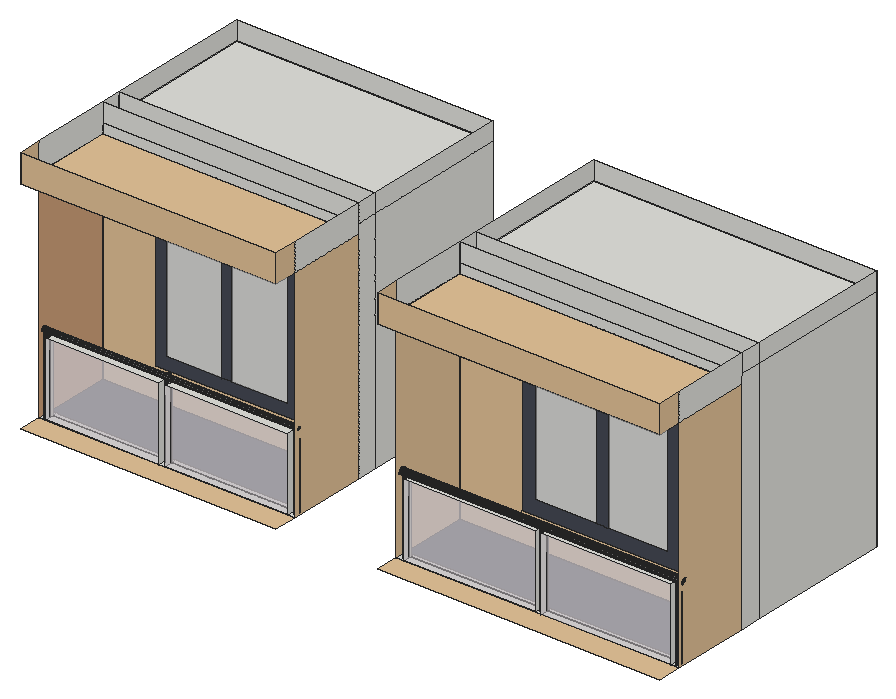
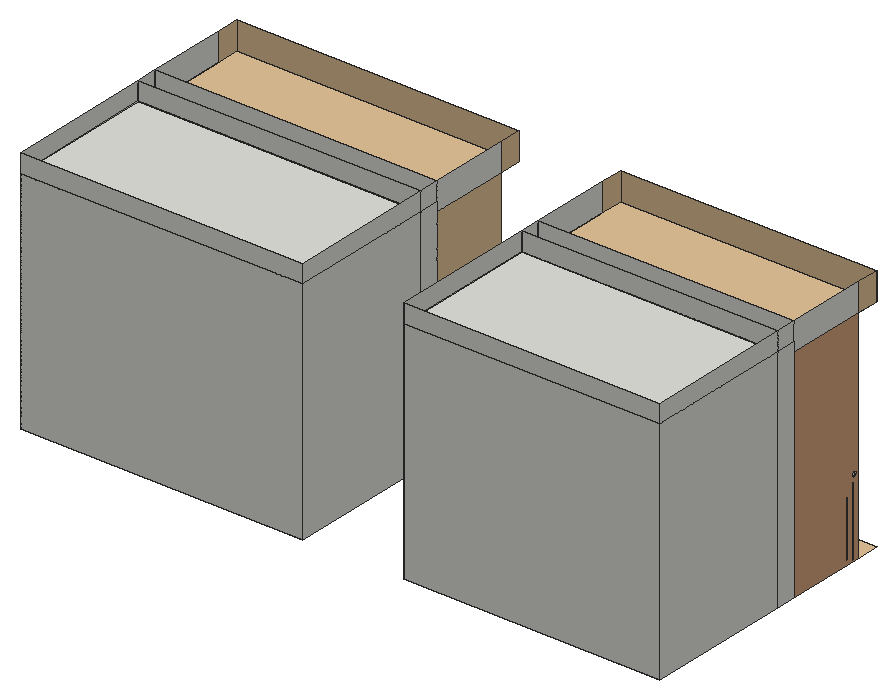
# SketchUp Ruby script. Lengths in inches.
U = 1.inch
M = Sketchup.active_model
def pt(a) = Geom::Point3d.new(a.map { |v| v * U })
def face(e, loops, mat)
  f = e.add_face(loops[0].map { |a| pt(a) })
  loops[1..].each { |l| e.add_face(l.map { |a| pt(a) }).erase! }
  f.material = f.back_material = mat if mat
  f
end
# faces: each face lists its corners as indices into pts; further lists are holes
def faces(e, pts, list, mat = nil) = list.each { |f| face(e, (f[0].is_a?(Array) ? f : [f]).map { |l| l.map { |i| pts[i] } }, mat) }
# xy, xz, yz: faces in a plane at the given z, y or x. An outline is a flat list of corners, or four numbers for a rectangle; further outlines are holes
def ring(l) = l.size == 4 ? [[l[0], l[1]], [l[2], l[1]], [l[2], l[3]], [l[0], l[3]]] : l.each_slice(2).to_a
def flat(e, list, mat, &to3) = list.each { |f| face(e, (f[0].is_a?(Array) ? f : [f]).map { |l| ring(l).map { |u, v| to3.(u, v) } }, mat) }
def xy(e, z, list, mat = nil) = flat(e, list, mat) { |x, y| [x, y, z] }
def xz(e, y, list, mat = nil) = flat(e, list, mat) { |x, z| [x, y, z] }
def yz(e, x, list, mat = nil) = flat(e, list, mat) { |y, z| [x, y, z] }
def lines(e, pts, list) = list.each { |a, b| e.add_line(pt(pts[a]), pt(pts[b])) }
# prism: a flat outline (further loops are holes) pulled along v
def prism(e, loops, v, mat = nil)
  f = face(e, loops, mat); d = Geom::Vector3d.new(v.map { |x| x * U })
  f.pushpull(f.normal.samedirection?(d) ? d.length : -d.length)
end
def box(e, o, s, mat = nil) = prism(e, [[o, [o[0] + s[0], o[1], o[2]], [o[0] + s[0], o[1] + s[1], o[2]], [o[0], o[1] + s[1], o[2]]]], [0, 0, s[2]], mat)
def at(x, y, z, deg = 0) = Geom::Transformation.translation(pt([x, y, z])) * Geom::Transformation.rotation(ORIGIN, Z_AXIS, deg.degrees)
def axes(o, x, y, z) = Geom::Transformation.new([*x, 0, *y, 0, *z, 0, *pt(o).to_a, 1])
def part(name) = M.definitions.add(name)
# library, detail: a bought-in or finely detailed component or shape, given as its bounding box
def library(name, o, s) = part(name).tap { |d| box(d.entities, o, s) }
def detail(e, o, s) = box(e.add_group.entities, o, s)
def put(e, d, t, mat = nil) = e.add_instance(d, t).tap { |i| i.material = mat if mat }
def group(e, t, mat = nil) = e.add_group.tap { |g| g.transformation = t; g.material = mat if mat }.entities
root = M.entities
M.materials.add("[0035_Tan]").color = [229, 196, 153]
M.materials.add("[Cladding Siding Tan]").color = [211, 164, 124]
M.materials.add("[Color M05]").color = [114, 114, 114]
M.materials.add("[Formica Laminate Dark]").color = [70, 74, 84]
M.materials.add("[Suede Blue]").color = [50, 57, 70]
M.materials.add("[Translucent Glass Gray]").color = [214, 214, 214]
M.materials["[Translucent Glass Gray]"].alpha = 0.5
M.materials.add("[Translucent Glass Safety]1").color = [244, 237, 242]
M.materials["[Translucent Glass Safety]1"].alpha = 0.5
xy(root,524.8125,[[[225.05,423.82,230.94,436.91],[228.4375,426.02,227.84,426.1,227.28,426.33,226.8,426.7,226.4375,427.18,226.2,427.73,226.125,428.33,226.2,428.93,226.4375,429.49,226.8,429.97,227.28,430.33,227.84,430.57,228.4375,430.64,229.04,430.57,229.59,430.33,230.07,429.97,230.44,429.49,230.67,428.93,230.75,428.33,230.67,427.73,230.44,427.18,230.07,426.7,229.59,426.33,229.04,426.1]],[230.94,423.82,335.79,431.96],[[335.79,423.82,340.97,436.91],[338.4375,428.08,337.84,428.16,337.28,428.39,336.8,428.76,336.4375,429.24,336.2,429.8,336.125,430.39,336.2,430.99,336.4375,431.55,336.8,432.03,337.28,432.4,337.84,432.63,338.4375,432.71,339.04,432.63,339.59,432.4,340.07,432.03,340.44,431.55,340.67,430.99,340.75,430.39,340.67,429.8,340.44,429.24,340.07,428.76,339.59,428.39,339.04,428.16]],[340.97,423.82,454.47,431.96],[[454.47,423.82,460.75,436.91],[457,428.08,456.4,428.16,455.84,428.39,455.37,428.76,455,429.24,454.77,429.8,454.6875,430.39,454.77,430.99,455,431.55,455.37,432.03,455.84,432.4,456.4,432.63,457,432.71,457.6,432.63,458.16,432.4,458.64,432.03,459,431.55,459.23,430.99,459.3125,430.39,459.23,429.8,459,429.24,458.64,428.76,458.16,428.39,457.6,428.16]],
  [[553.875,423.82,561.125,435],[558.4,426.88,557.77,426.96,557.1875,427.2,556.68,427.59,556.29,428.1,556.05,428.68,555.97,429.32,556.05,429.95,556.29,430.53,556.68,431.04,557.1875,431.43,557.77,431.67,558.4,431.75,559.04,431.67,559.625,431.43,560.13,431.04,560.52,430.53,560.76,429.95,560.84,429.32,560.76,428.68,560.52,428.1,560.13,427.59,559.625,427.2,559.04,426.96]],[561.125,423.82,682.3125,431.3],[[682.3125,423.82,687.5625,435],[684.97,426.88,684.34,426.96,683.75,427.2,683.24,427.59,682.86,428.1,682.61,428.68,682.53,429.32,682.61,429.95,682.86,430.53,683.24,431.04,683.75,431.43,684.34,431.67,684.97,431.75,685.6,431.67,686.1875,431.43,686.69,431.04,687.08,430.53,687.32,429.95,687.4,429.32,687.32,428.68,687.08,428.1,686.69,427.59,686.1875,427.2,685.6,426.96]],[687.5625,423.82,807.1,431.3],[[807.1,423.82,814,435],[809.9,426.88,809.27,426.96,808.6875,427.2,808.18,427.59,807.79,428.1,807.55,428.68,807.47,429.32,807.55,429.95,807.79,430.53,808.18,431.04,808.6875,431.43,809.27,431.67,809.9,431.75,810.54,431.67,811.125,431.43,811.63,431.04,812.02,430.53,812.26,429.95,812.34,429.32,812.26,428.68,812.02,428.1,811.63,427.59,811.125,427.2,810.54,426.96]],
  [228.4375,426.02,227.84,426.1,227.28,426.33,226.8,426.7,226.4375,427.18,226.2,427.73,226.125,428.33,226.2,428.93,226.4375,429.49,226.8,429.97,227.28,430.33,227.84,430.57,228.4375,430.64,229.04,430.57,229.59,430.33,230.07,429.97,230.44,429.49,230.67,428.93,230.75,428.33,230.67,427.73,230.44,427.18,230.07,426.7,229.59,426.33,229.04,426.1],[558.4,426.88,557.77,426.96,557.1875,427.2,556.68,427.59,556.29,428.1,556.05,428.68,555.97,429.32,556.05,429.95,556.29,430.53,556.68,431.04,557.1875,431.43,557.77,431.67,558.4,431.75,559.04,431.67,559.625,431.43,560.13,431.04,560.52,430.53,560.76,429.95,560.84,429.32,560.76,428.68,560.52,428.1,560.13,427.59,559.625,427.2,559.04,426.96],[684.97,426.88,684.34,426.96,683.75,427.2,683.24,427.59,682.86,428.1,682.61,428.68,682.53,429.32,682.61,429.95,682.86,430.53,683.24,431.04,683.75,431.43,684.34,431.67,684.97,431.75,685.6,431.67,686.1875,431.43,686.69,431.04,687.08,430.53,687.32,429.95,687.4,429.32,687.32,428.68,687.08,428.1,686.69,427.59,686.1875,427.2,685.6,426.96],[809.9,426.88,809.27,426.96,808.6875,427.2,808.18,427.59,807.79,428.1,807.55,428.68,807.47,429.32,807.55,429.95,807.79,430.53,808.18,431.04,808.6875,431.43,809.27,431.67,809.9,431.75,810.54,431.67,811.125,431.43,811.63,431.04,812.02,430.53,812.26,429.95,812.34,429.32,812.26,428.68,812.02,428.1,811.63,427.59,811.125,427.2,810.54,426.96],[338.4375,428.08,337.84,428.16,337.28,428.39,336.8,428.76,336.4375,429.24,336.2,429.8,336.125,430.39,336.2,430.99,336.4375,431.55,336.8,432.03,337.28,432.4,337.84,432.63,338.4375,432.71,339.04,432.63,339.59,432.4,340.07,432.03,340.44,431.55,340.67,430.99,340.75,430.39,340.67,429.8,340.44,429.24,340.07,428.76,339.59,428.39,339.04,428.16],
  [457,428.08,456.4,428.16,455.84,428.39,455.37,428.76,455,429.24,454.77,429.8,454.6875,430.39,454.77,430.99,455,431.55,455.37,432.03,455.84,432.4,456.4,432.63,457,432.71,457.6,432.63,458.16,432.4,458.64,432.03,459,431.55,459.23,430.99,459.3125,430.39,459.23,429.8,459,429.24,458.64,428.76,458.16,428.39,457.6,428.16],[561.125,431.3,682.3125,435],[687.5625,431.3,807.1,435],[230.94,431.96,335.79,436.91],[340.97,431.96,454.47,436.91],
  [225.05,496.86,460.75,515.85],[553.875,496.86,814,515.85],[225.05,515.85,460.75,651.39],[553.875,515.85,814,651.39]])
xy(root,524.8125,[[225.05,402.38,460.75,423.82],[553.875,402.38,814,423.82]],"[0035_Tan]")
xy(root,524.8125,[[553.875,435,814,496.86],[225.05,436.91,460.75,496.86]],"[Suede Blue]")
xy(root,592.1875,[[230.94,423.82,335.79,431.96],[340.97,423.82,454.47,431.96],[561.125,423.82,682.3125,431.3],[687.5625,423.82,807.1,431.3]])
xy(root,593.42,[[684.97,426.88,685.6,426.96,686.1875,427.2,686.69,427.59,687.08,428.1,687.32,428.68,687.4,429.32,687.32,429.95,687.08,430.53,686.69,431.04,686.1875,431.43,685.6,431.67,684.97,431.75,684.34,431.67,683.75,431.43,683.24,431.04,682.86,430.53,682.61,429.95,682.53,429.32,682.61,428.68,682.86,428.1,683.24,427.59,683.75,427.2,684.34,426.96]])
xy(root,594.16,[[558.4,426.88,559.04,426.96,559.625,427.2,560.13,427.59,560.52,428.1,560.76,428.68,560.84,429.32,560.76,429.95,560.52,430.53,560.13,431.04,559.625,431.43,559.04,431.67,558.4,431.75,557.77,431.67,557.1875,431.43,556.68,431.04,556.29,430.53,556.05,429.95,555.97,429.32,556.05,428.68,556.29,428.1,556.68,427.59,557.1875,427.2,557.77,426.96],[809.9,426.88,810.54,426.96,811.125,427.2,811.63,427.59,812.02,428.1,812.26,428.68,812.34,429.32,812.26,429.95,812.02,430.53,811.63,431.04,811.125,431.43,810.54,431.67,809.9,431.75,809.27,431.67,808.6875,431.43,808.18,431.04,807.79,430.53,807.55,429.95,807.47,429.32,807.55,428.68,807.79,428.1,808.18,427.59,808.6875,427.2,809.27,426.96]])
xy(root,594.5625,[[457,428.08,457.6,428.16,458.16,428.39,458.64,428.76,459,429.24,459.23,429.8,459.3125,430.39,459.23,430.99,459,431.55,458.64,432.03,458.16,432.4,457.6,432.63,457,432.71,456.4,432.63,455.84,432.4,455.37,432.03,455,431.55,454.77,430.99,454.6875,430.39,454.77,429.8,455,429.24,455.37,428.76,455.84,428.39,456.4,428.16]])
xy(root,596.5625,[[228.4375,426.02,229.04,426.1,229.59,426.33,230.07,426.7,230.44,427.18,230.67,427.73,230.75,428.33,230.67,428.93,230.44,429.49,230.07,429.97,229.59,430.33,229.04,430.57,228.4375,430.64,227.84,430.57,227.28,430.33,226.8,429.97,226.4375,429.49,226.2,428.93,226.125,428.33,226.2,427.73,226.4375,427.18,226.8,426.7,227.28,426.33,227.84,426.1]])
xy(root,597.06,[[338.4375,428.08,339.04,428.16,339.59,428.39,340.07,428.76,340.44,429.24,340.67,429.8,340.74,430.35,336.13,430.35,336.2,429.8,336.4375,429.24,336.8,428.76,337.28,428.39,337.84,428.16],[336.13,430.35,340.74,430.35,340.75,430.39,340.67,430.99,340.44,431.55,340.07,432.03,339.59,432.4,339.04,432.63,338.4375,432.71,337.84,432.63,337.28,432.4,336.8,432.03,336.4375,431.55,336.2,430.99,336.125,430.39]])
xy(root,727.0625,[[225.05,402.38,460.75,496.86],[553.875,402.38,814,496.86]],"[0035_Tan]")
xy(root,735.5,[[225.05,496.86,460.75,515.85],[553.875,496.86,814,515.85],[225.05,515.85,460.75,651.39],[553.875,515.85,814,651.39]])
xz(root,402.38,[[225.05,727.0625,460.75,752.6875],[553.875,727.0625,814,752.6875]],"[0035_Tan]")
xz(root,423.82,[[230.94,524.8125,335.79,592.1875],[340.97,524.8125,454.47,592.1875],[561.125,524.8125,682.3125,592.1875],[687.5625,524.8125,807.1,592.1875]],"[Translucent Glass Safety]1")
xz(root,431.3,[[561.125,524.8125,682.3125,592.1875],[687.5625,524.8125,807.1,592.1875]],"[Translucent Glass Safety]1")
xz(root,431.96,[[230.94,524.8125,335.79,592.1875],[340.97,524.8125,454.47,592.1875]],"[Translucent Glass Safety]1")
xz(root,496.86,[[225.05,727.0625,460.75,735.5],[553.875,727.0625,814,735.5],[225.05,735.5,460.75,752.6875],[553.875,735.5,814,752.6875]])
xz(root,496.86,[[[225.05,524.8125,460.75,727.0625],[273.85,552.86,406.72,707.17]],[[553.875,524.8125,814,727.0625],[611.02,551.65,759.09,708.4]]],"[0035_Tan]")
xz(root,496.86,[[[611.02,551.65,759.09,708.4],[624.18,564.81,745.92,695.24]],[[273.85,552.86,406.72,707.17],[284.63,563.64,395.95,696.39]],[335.36,563.64,344.53,696.39],[679.95,564.81,691.15,695.24]],"[Formica Laminate Dark]")
xz(root,496.86,[[284.63,563.64,335.36,696.39],[344.53,563.64,395.95,696.39],[624.18,564.81,679.95,695.24],[691.15,564.81,745.92,695.24]],"[Translucent Glass Gray]")
xz(root,515.85,[[225.05,524.8125,460.75,735.5],[553.875,524.8125,814,735.5],[225.05,735.5,460.75,752.6875],[553.875,735.5,814,752.6875]])
xz(root,651.39,[[225.05,524.8125,460.75,735.5],[553.875,524.8125,814,735.5],[225.05,735.5,460.75,752.6875],[553.875,735.5,814,752.6875]])
yz(root,225.05,[[496.86,524.8125,515.85,735.5],[515.85,524.8125,651.39,735.5],[428.41,594.54,427.9,594.61,427.41,594.81,427,595.13,426.68,595.54,426.48,596.02,426.41,596.54,426.48,597.06,426.68,597.54,427,597.96,427.41,598.27,427.9,598.47,428.41,598.54,428.93,598.47,429.41,598.27,429.83,597.96,430.15,597.54,430.35,597.06,430.41,596.54,430.35,596.02,430.15,595.54,429.83,595.13,429.41,594.81,428.93,594.61],[423.82,727.0625,496.86,752.6875],[496.86,735.5,515.85,752.6875],
  [515.85,735.5,651.39,752.6875]])
yz(root,225.05,[[402.38,727.0625,423.82,752.6875]],"[0035_Tan]")
yz(root,225.05,[[[423.82,524.8125,496.86,727.0625],[428.41,594.54,427.9,594.61,427.41,594.81,427,595.13,426.68,595.54,426.48,596.02,426.41,596.54,426.48,597.06,426.68,597.54,427,597.96,427.41,598.27,427.9,598.47,428.41,598.54,428.93,598.47,429.41,598.27,429.83,597.96,430.15,597.54,430.35,597.06,430.41,596.54,430.35,596.02,430.15,595.54,429.83,595.13,429.41,594.81,428.93,594.61]]],"[Cladding Siding Tan]")
yz(root,230.94,[[423.82,524.8125,431.96,592.1875]])
yz(root,335.79,[[423.82,524.8125,431.96,592.1875]])
yz(root,340.97,[[423.82,524.8125,431.96,592.1875]])
yz(root,454.47,[[423.82,524.8125,431.96,592.1875]])
yz(root,460.75,[[496.86,524.8125,515.85,735.5],[515.85,524.8125,651.39,735.5],[423.82,727.0625,496.86,752.6875],[496.86,735.5,515.85,752.6875],[515.85,735.5,651.39,752.6875]])
yz(root,460.75,[[[423.82,524.8125,496.86,727.0625],[428.41,594.54,428.93,594.61,429.41,594.81,429.83,595.13,430.15,595.54,430.35,596.02,430.41,596.54,430.35,597.06,430.15,597.54,429.83,597.96,429.41,598.27,428.93,598.47,428.41,598.54,427.9,598.47,427.41,598.27,427,597.96,426.68,597.54,426.48,597.06,426.41,596.54,426.48,596.02,426.68,595.54,427,595.13,427.41,594.81,427.9,594.61]],[402.38,727.0625,423.82,752.6875]],"[0035_Tan]")
yz(root,553.875,[[496.86,524.8125,515.85,735.5],[515.85,524.8125,651.39,735.5],[429.625,591.29,428.88,591.38,428.1875,591.67,427.59,592.13,427.14,592.72,426.85,593.42,426.75,594.16,426.85,594.9,427.14,595.6,427.59,596.19,428.1875,596.65,428.88,596.9375,429.625,597.04,430.37,596.9375,431.0625,596.65,431.66,596.19,432.12,595.6,432.4,594.9,432.5,594.16,432.4,593.42,432.12,592.72,431.66,592.13,431.0625,591.67,430.37,591.38],[423.82,727.0625,496.86,752.6875],[496.86,735.5,515.85,752.6875],
  [515.85,735.5,651.39,752.6875]])
yz(root,553.875,[[[423.82,524.8125,496.86,727.0625],[429.625,591.29,428.88,591.38,428.1875,591.67,427.59,592.13,427.14,592.72,426.85,593.42,426.75,594.16,426.85,594.9,427.14,595.6,427.59,596.19,428.1875,596.65,428.88,596.9375,429.625,597.04,430.37,596.9375,431.0625,596.65,431.66,596.19,432.12,595.6,432.4,594.9,432.5,594.16,432.4,593.42,432.12,592.72,431.66,592.13,431.0625,591.67,430.37,591.38]],[402.38,727.0625,423.82,752.6875]],"[0035_Tan]")
yz(root,561.125,[[423.82,524.8125,431.3,592.1875]])
yz(root,682.3125,[[423.82,524.8125,431.3,592.1875]])
yz(root,687.5625,[[423.82,524.8125,431.3,592.1875]])
yz(root,807.1,[[423.82,524.8125,431.3,592.1875]])
yz(root,814,[[496.86,524.8125,515.85,735.5],[515.85,524.8125,651.39,735.5],[423.82,727.0625,496.86,752.6875],[496.86,735.5,515.85,752.6875],[515.85,735.5,651.39,752.6875]])
yz(root,814,[[[423.82,524.8125,496.86,727.0625],[429.625,591.29,430.37,591.38,431.0625,591.67,431.66,592.13,432.12,592.72,432.4,593.42,432.5,594.16,432.4,594.9,432.12,595.6,431.66,596.19,431.0625,596.65,430.37,596.9375,429.625,597.04,428.88,596.9375,428.1875,596.65,427.59,596.19,427.14,595.6,426.85,594.9,426.75,594.16,426.85,593.42,427.14,592.72,427.59,592.13,428.1875,591.67,428.88,591.38]],[402.38,727.0625,423.82,752.6875]],"[0035_Tan]")
p = [[227.84,426.1,524.8125],[228.4375,426.02,524.8125],[228.4375,426.02,596.5625],[227.84,426.1,596.5625],[229.04,426.1,524.8125],[229.04,426.1,596.5625],
  [227.28,426.33,524.8125],[227.28,426.33,596.5625],[229.59,426.33,524.8125],[229.59,426.33,596.5625],[226.8,426.7,524.8125],[226.8,426.7,596.5625],
  [230.07,426.7,524.8125],[230.07,426.7,596.5625],[226.4375,427.18,524.8125],[226.4375,427.18,596.5625],[230.44,427.18,524.8125],[230.44,427.18,596.5625],
  [557.77,426.96,524.8125],[558.4,426.88,524.8125],[558.4,426.88,594.16],[557.77,426.96,594.16],[559.04,426.96,524.8125],[559.04,426.96,594.16],
  [684.34,426.96,524.8125],[684.97,426.88,524.8125],[684.97,426.88,593.42],[684.34,426.96,593.42],[685.6,426.96,524.8125],[685.6,426.96,593.42],
  [809.27,426.96,524.8125],[809.9,426.88,524.8125],[809.9,426.88,594.16],[809.27,426.96,594.16],[810.54,426.96,524.8125],[810.54,426.96,594.16],
  [557.1875,427.2,524.8125],[557.1875,427.2,594.16],[559.625,427.2,524.8125],[559.625,427.2,594.16],[683.75,427.2,524.8125],[683.75,427.2,593.42],
  [686.1875,427.2,524.8125],[686.1875,427.2,593.42],[808.6875,427.2,524.8125],[808.6875,427.2,594.16],[811.125,427.2,524.8125],[811.125,427.2,594.16],
  [226.2,427.73,524.8125],[226.2,427.73,596.5625],[230.67,427.73,524.8125],[230.67,427.73,596.5625],[556.68,427.59,524.8125],[556.68,427.59,594.16],
  [556.68,427.59,592.13],[560.13,427.59,524.8125],[560.13,427.59,592.13],[560.13,427.59,594.16],[683.24,427.59,524.8125],[683.24,427.59,593.42],
  [683.24,427.59,592.13],[686.69,427.59,524.8125],[686.69,427.59,592.13],[686.69,427.59,593.42],[808.18,427.59,524.8125],[808.18,427.59,594.16],
  [808.18,427.59,592.13],[811.63,427.59,524.8125],[811.63,427.59,592.13],[811.63,427.59,594.16],[556.29,428.1,524.8125],[556.29,428.1,594.16],
  [560.52,428.1,524.8125],[560.52,428.1,594.16],[682.86,428.1,524.8125],[682.86,428.1,593.42],[687.08,428.1,524.8125],[687.08,428.1,593.42],
  [807.79,428.1,524.8125],[807.79,428.1,594.16],[812.02,428.1,524.8125],[812.02,428.1,594.16],[226.125,428.33,524.8125],[226.125,428.33,596.5625],
  [230.75,428.33,524.8125],[230.75,428.33,596.5625],[337.84,428.16,524.8125],[338.4375,428.08,524.8125],[338.4375,428.08,597.06],[337.84,428.16,597.06],
  [339.04,428.16,524.8125],[339.04,428.16,597.06],[456.4,428.16,524.8125],[457,428.08,524.8125],[457,428.08,594.5625],[456.4,428.16,594.5625],
  [457.6,428.16,524.8125],[457.6,428.16,594.5625],[556.05,428.68,524.8125],[556.05,428.68,594.16],[560.76,428.68,524.8125],[560.76,428.68,594.16],
  [682.61,428.68,524.8125],[682.61,428.68,593.42],[687.32,428.68,524.8125],[687.32,428.68,593.42],[807.55,428.68,524.8125],[807.55,428.68,594.16],
  [812.26,428.68,524.8125],[812.26,428.68,594.16],[337.28,428.39,524.8125],[337.28,428.39,597.06],[339.59,428.39,524.8125],[339.59,428.39,597.06],
  [455.84,428.39,524.8125],[455.84,428.39,594.5625],[458.16,428.39,524.8125],[458.16,428.39,594.5625],[226.2,428.93,524.8125],[226.2,428.93,596.5625],
  [226.2,428.93,594.61],[230.67,428.93,524.8125],[230.67,428.93,594.61],[230.67,428.93,596.5625],[336.8,428.76,524.8125],[336.8,428.76,597.06],
  [340.07,428.76,524.8125],[340.07,428.76,597.06],[455.37,428.76,524.8125],[455.37,428.76,594.5625],[458.64,428.76,524.8125],[458.64,428.76,594.5625],
  [555.97,429.32,524.8125],[555.97,429.32,594.16],[560.84,429.32,524.8125],[560.84,429.32,594.16],[682.53,429.32,524.8125],[682.53,429.32,593.42],
  [687.4,429.32,524.8125],[687.4,429.32,593.42],[807.47,429.32,524.8125],[807.47,429.32,594.16],[812.34,429.32,524.8125],[812.34,429.32,594.16],
  [336.4375,429.24,524.8125],[336.4375,429.24,597.06],[340.44,429.24,524.8125],[340.44,429.24,597.06],[455,429.24,524.8125],[455,429.24,594.5625],
  [459,429.24,524.8125],[459,429.24,594.5625],[226.4375,429.49,524.8125],[226.4375,429.49,596.5625],[230.44,429.49,524.8125],[230.44,429.49,596.5625],
  [336.2,429.8,524.8125],[336.2,429.8,597.06],[340.67,429.8,524.8125],[340.67,429.8,597.06],[454.77,429.8,524.8125],[454.77,429.8,594.5625],
  [459.23,429.8,524.8125],[459.23,429.8,594.5625],[556.05,429.95,524.8125],[556.05,429.95,594.16],[560.76,429.95,524.8125],[560.76,429.95,594.16],
  [682.61,429.95,524.8125],[682.61,429.95,593.42],[687.32,429.95,524.8125],[687.32,429.95,593.42],[807.55,429.95,524.8125],[807.55,429.95,594.16],
  [812.26,429.95,524.8125],[812.26,429.95,594.16],[226.8,429.97,524.8125],[226.8,429.97,596.5625],[230.07,429.97,524.8125],[230.07,429.97,596.5625],
  [336.125,430.39,524.8125],[336.13,430.35,597.06],[336.125,430.39,597.06],[340.75,430.39,524.8125],[340.75,430.39,597.06],[340.74,430.35,597.06],
  [454.6875,430.39,524.8125],[454.6875,430.39,594.5625],[459.3125,430.39,524.8125],[459.3125,430.39,594.5625],[556.29,430.53,524.8125],[556.29,430.53,594.16],
  [560.52,430.53,524.8125],[560.52,430.53,594.16],[682.86,430.53,524.8125],[682.86,430.53,593.42],[687.08,430.53,524.8125],[687.08,430.53,593.42],
  [807.79,430.53,524.8125],[807.79,430.53,594.16],[812.02,430.53,524.8125],[812.02,430.53,594.16],[227.28,430.33,524.8125],[227.28,430.33,596.5625],
  [229.59,430.33,524.8125],[229.59,430.33,596.5625],[227.84,430.57,524.8125],[227.84,430.57,596.5625],[229.04,430.57,524.8125],[229.04,430.57,596.5625],
  [336.2,430.99,524.8125],[336.2,430.99,597.06],[340.67,430.99,524.8125],[340.67,430.99,597.06],[454.77,430.99,524.8125],[454.77,430.99,594.5625],
  [459.23,430.99,524.8125],[459.23,430.99,594.5625],[556.68,431.04,524.8125],[556.68,431.04,594.16],[560.13,431.04,524.8125],[560.13,431.04,594.16],
  [683.24,431.04,524.8125],[683.24,431.04,593.42],[686.69,431.04,524.8125],[686.69,431.04,593.42],[808.18,431.04,524.8125],[808.18,431.04,594.16],
  [811.63,431.04,524.8125],[811.63,431.04,594.16],[228.4375,430.64,524.8125],[228.4375,430.64,596.5625],[336.4375,431.55,524.8125],[336.4375,431.55,597.06],
  [340.44,431.55,524.8125],[340.44,431.55,597.06],[455,431.55,524.8125],[455,431.55,594.5625],[459,431.55,524.8125],[459,431.55,594.5625],
  [557.1875,431.43,524.8125],[557.1875,431.43,594.16],[559.625,431.43,524.8125],[559.625,431.43,594.16],[683.75,431.43,524.8125],[683.75,431.43,593.42],
  [686.1875,431.43,524.8125],[686.1875,431.43,593.42],[808.6875,431.43,524.8125],[808.6875,431.43,594.16],[811.125,431.43,524.8125],[811.125,431.43,594.16],
  [557.77,431.67,524.8125],[557.77,431.67,594.16],[559.04,431.67,524.8125],[559.04,431.67,594.16],[684.34,431.67,524.8125],[684.34,431.67,593.42],
  [685.6,431.67,524.8125],[685.6,431.67,593.42],[809.27,431.67,524.8125],[809.27,431.67,594.16],[810.54,431.67,524.8125],[810.54,431.67,594.16],
  [336.8,432.03,524.8125],[336.8,432.03,597.06],[340.07,432.03,524.8125],[340.07,432.03,597.06],[455.37,432.03,524.8125],[455.37,432.03,594.5625],
  [458.64,432.03,524.8125],[458.64,432.03,594.5625],[558.4,431.75,524.8125],[558.4,431.75,594.16],[684.97,431.75,524.8125],[684.97,431.75,593.42],
  [809.9,431.75,524.8125],[809.9,431.75,594.16],[337.28,432.4,524.8125],[337.28,432.4,597.06],[339.59,432.4,524.8125],[339.59,432.4,597.06],
  [455.84,432.4,524.8125],[455.84,432.4,594.5625],[458.16,432.4,524.8125],[458.16,432.4,594.5625],[337.84,432.63,524.8125],[337.84,432.63,597.06],
  [339.04,432.63,524.8125],[339.04,432.63,597.06],[456.4,432.63,524.8125],[456.4,432.63,594.5625],[457.6,432.63,524.8125],[457.6,432.63,594.5625],
  [338.4375,432.71,524.8125],[338.4375,432.71,597.06],[457,432.71,524.8125],[457,432.71,594.5625],[553.875,428.88,591.38],[553.875,429.625,591.29],
  [814,429.625,591.29],[814,428.88,591.38],[553.875,430.37,591.38],[814,430.37,591.38],[553.875,428.1875,591.67],[814,428.1875,591.67],
  [553.875,431.0625,591.67],[814,431.0625,591.67],[553.875,427.59,592.13],[814,427.59,592.13],[553.875,431.66,592.13],[814,431.66,592.13],
  [553.875,427.14,592.72],[814,427.14,592.72],[553.875,432.12,592.72],[814,432.12,592.72],[553.875,426.85,593.42],[814,426.85,593.42],
  [553.875,432.4,593.42],[814,432.4,593.42],[553.875,426.75,594.16],[814,426.75,594.16],[553.875,432.5,594.16],[814,432.5,594.16],
  [553.875,426.85,594.9],[814,426.85,594.9],[553.875,432.4,594.9],[814,432.4,594.9],[225.05,427.9,594.61],[225.05,428.41,594.54],
  [460.75,428.41,594.54],[460.75,427.9,594.61],[225.05,428.93,594.61],[460.75,428.93,594.61],[225.05,427.41,594.81],[460.75,427.41,594.81],
  [225.05,429.41,594.81],[460.75,429.41,594.81],[225.05,427,595.13],[460.75,427,595.13],[225.05,429.83,595.13],[460.75,429.83,595.13],
  [553.875,427.14,595.6],[814,427.14,595.6],[553.875,432.12,595.6],[814,432.12,595.6],[225.05,426.68,595.54],[460.75,426.68,595.54],
  [225.05,430.15,595.54],[460.75,430.15,595.54],[225.05,426.48,596.02],[460.75,426.48,596.02],[225.05,430.35,596.02],[460.75,430.35,596.02],
  [553.875,427.59,596.19],[814,427.59,596.19],[553.875,431.66,596.19],[814,431.66,596.19],[225.05,426.41,596.54],[460.75,426.41,596.54],
  [225.05,430.41,596.54],[460.75,430.41,596.54],[553.875,428.1875,596.65],[814,428.1875,596.65],[553.875,431.0625,596.65],[814,431.0625,596.65],
  [225.05,426.48,597.06],[460.75,426.48,597.06],[225.05,430.35,597.06],[460.75,430.35,597.06],[553.875,428.88,596.9375],[814,428.88,596.9375],
  [553.875,430.37,596.9375],[814,430.37,596.9375],[553.875,429.625,597.04],[814,429.625,597.04],[225.05,426.68,597.54],[460.75,426.68,597.54],
  [225.05,430.15,597.54],[460.75,430.15,597.54],[225.05,427,597.96],[460.75,427,597.96],[225.05,429.83,597.96],[460.75,429.83,597.96],
  [225.05,427.41,598.27],[460.75,427.41,598.27],[225.05,429.41,598.27],[460.75,429.41,598.27],[225.05,427.9,598.47],[460.75,427.9,598.47],
  [225.05,428.93,598.47],[460.75,428.93,598.47],[225.05,428.41,598.54],[460.75,428.41,598.54]]
faces(root,p,[[0,1,2,3],[1,4,5,2],[6,0,3,7],[4,8,9,5],[10,6,7,11],[8,12,13,9],[14,10,11,15],[12,16,17,13],
  [18,19,20,21],[19,22,23,20],[24,25,26,27],[25,28,29,26],[30,31,32,33],[31,34,35,32],[36,18,21,37],[22,38,39,23],
  [40,24,27,41],[28,42,43,29],[44,30,33,45],[34,46,47,35],[48,14,15,49],[16,50,51,17],[52,36,37,53,54],[38,55,56,57,39],
  [58,40,41,59,60],[42,61,62,63,43],[64,44,45,65,66],[46,67,68,69,47],[70,52,54,53,71],[55,72,73,57,56],[74,58,60,59,75],[61,76,77,63,62],
  [78,64,66,65,79],[67,80,81,69,68],[82,48,49,83],[50,84,85,51],[86,87,88,89],[87,90,91,88],[92,93,94,95],[93,96,97,94],
  [98,70,71,99],[72,100,101,73],[102,74,75,103],[76,104,105,77],[106,78,79,107],[80,108,109,81],[110,86,89,111],[90,112,113,91],
  [114,92,95,115],[96,116,117,97],[118,82,83,119,120],[84,121,122,123,85],[124,110,111,125],[112,126,127,113],[128,114,115,129],[116,130,131,117],
  [132,98,99,133],[100,134,135,101],[136,102,103,137],[104,138,139,105],[140,106,107,141],[108,142,143,109],[144,124,125,145],[126,146,147,127],
  [148,128,129,149],[130,150,151,131],[152,118,120,119,153],[121,154,155,123,122],[156,144,145,157],[146,158,159,147],[160,148,149,161],[150,162,163,151],
  [164,132,133,165],[134,166,167,135],[168,136,137,169],[138,170,171,139],[172,140,141,173],[142,174,175,143],[176,152,153,177],[154,178,179,155],
  [180,156,157,181,182],[158,183,184,185,159],[186,160,161,187],[162,188,189,163],[190,164,165,191],[166,192,193,167],[194,168,169,195],[170,196,197,171],
  [198,172,173,199],[174,200,201,175],[202,176,177,203],[178,204,205,179],[206,202,203,207],[204,208,209,205],[210,180,182,211],[183,212,213,184],
  [214,186,187,215],[188,216,217,189],[218,190,191,219],[192,220,221,193],[222,194,195,223],[196,224,225,197],[226,198,199,227],[200,228,229,201],
  [230,206,207,231],[208,230,231,209],[232,210,211,233],[212,234,235,213],[236,214,215,237],[216,238,239,217],[240,218,219,241],[220,242,243,221],
  [244,222,223,245],[224,246,247,225],[248,226,227,249],[228,250,251,229],[252,240,241,253],[242,254,255,243],[256,244,245,257],[246,258,259,247],
  [260,248,249,261],[250,262,263,251],[264,232,233,265],[234,266,267,235],[268,236,237,269],[238,270,271,239],[272,252,253,273],[254,272,273,255],
  [274,256,257,275],[258,274,275,259],[276,260,261,277],[262,276,277,263],[278,264,265,279],[266,280,281,267],[282,268,269,283],[270,284,285,271],
  [286,278,279,287],[280,288,289,281],[290,282,283,291],[284,292,293,285],[294,286,287,295],[288,294,295,289],[296,290,291,297],[292,296,297,293],
  [298,299,300,301],[299,302,303,300],[304,298,301,305],[302,306,307,303],[308,304,305,309,68,66,62,60,56,54],[306,310,311,307],[312,308,54,56,60,62,66,68,309,313],[310,314,315,311],
  [316,312,313,317],[314,318,319,315],[320,316,317,321],[318,322,323,319],[324,320,321,325],[322,326,327,323],[328,329,330,331],[329,332,120,122,333,330],
  [334,328,331,335],[332,336,337,333,122,120],[338,334,335,339],[336,340,341,337],[342,324,325,343],[326,344,345,327],[346,338,339,347],[340,348,349,341],
  [350,346,347,351],[348,352,353,349],[354,342,343,355],[344,356,357,345],[358,350,351,359],[352,360,361,353],[362,354,355,363],[356,364,365,357],
  [366,358,359,367],[360,368,181,185,369,361],[370,362,363,371],[364,372,373,365],[374,370,371,375],[372,374,375,373],[376,366,367,377],[368,378,379,369,185,181],
  [380,376,377,381],[378,382,383,379],[384,380,381,385],[382,386,387,383],[388,384,385,389],[386,390,391,387],[392,388,389,393],[390,392,393,391]],"[Color M05]")
